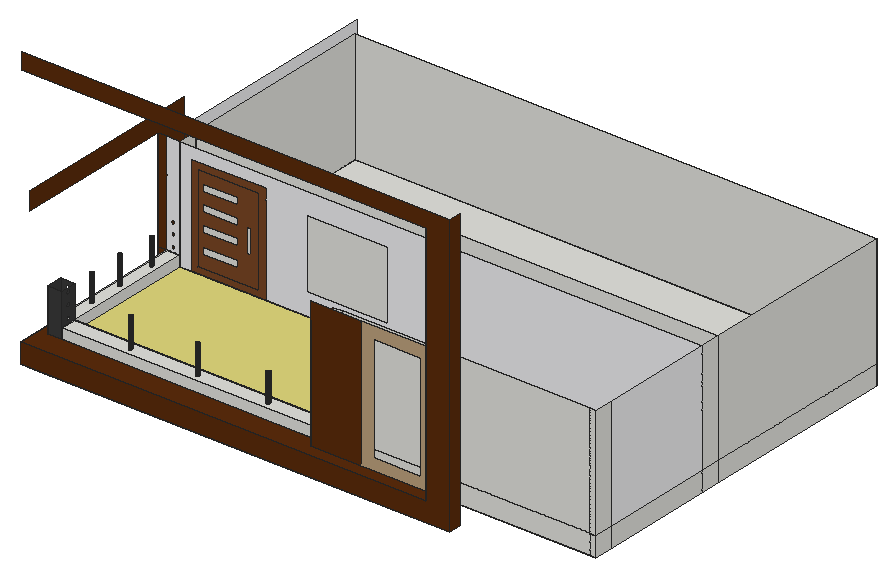
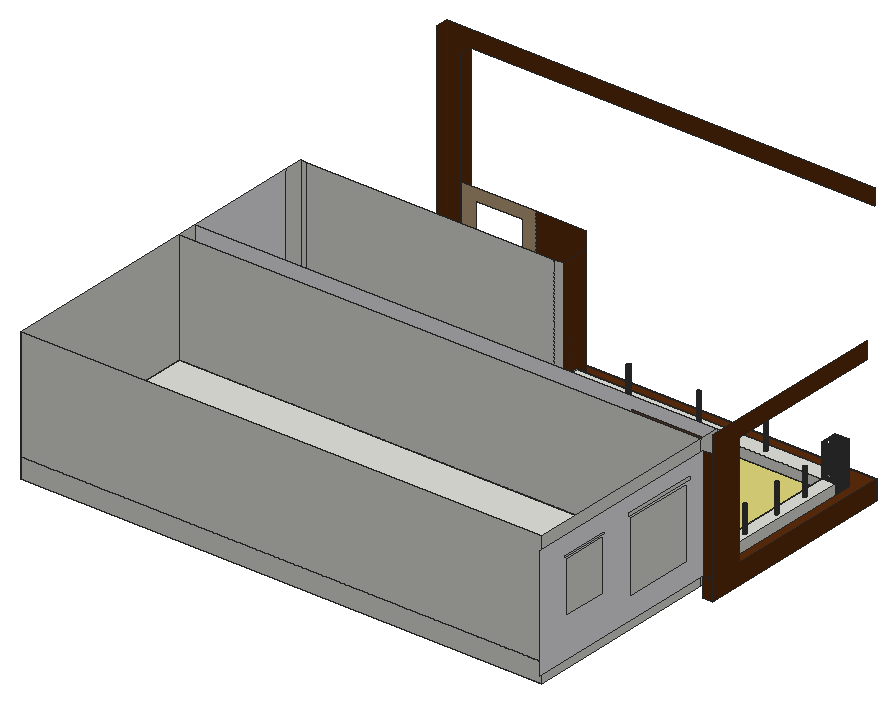
# SketchUp Ruby script. Lengths in inches.
U = 1.inch
M = Sketchup.active_model
def pt(a) = Geom::Point3d.new(a.map { |v| v * U })
def face(e, loops, mat)
  f = e.add_face(loops[0].map { |a| pt(a) })
  loops[1..].each { |l| e.add_face(l.map { |a| pt(a) }).erase! }
  f.material = f.back_material = mat if mat
  f
end
# faces: each face lists its corners as indices into pts; further lists are holes
def faces(e, pts, list, mat = nil) = list.each { |f| face(e, (f[0].is_a?(Array) ? f : [f]).map { |l| l.map { |i| pts[i] } }, mat) }
# xy, xz, yz: faces in a plane at the given z, y or x. An outline is a flat list of corners, or four numbers for a rectangle; further outlines are holes
def ring(l) = l.size == 4 ? [[l[0], l[1]], [l[2], l[1]], [l[2], l[3]], [l[0], l[3]]] : l.each_slice(2).to_a
def flat(e, list, mat, &to3) = list.each { |f| face(e, (f[0].is_a?(Array) ? f : [f]).map { |l| ring(l).map { |u, v| to3.(u, v) } }, mat) }
def xy(e, z, list, mat = nil) = flat(e, list, mat) { |x, y| [x, y, z] }
def xz(e, y, list, mat = nil) = flat(e, list, mat) { |x, z| [x, y, z] }
def yz(e, x, list, mat = nil) = flat(e, list, mat) { |y, z| [x, y, z] }
def lines(e, pts, list) = list.each { |a, b| e.add_line(pt(pts[a]), pt(pts[b])) }
# prism: a flat outline (further loops are holes) pulled along v
def prism(e, loops, v, mat = nil)
  f = face(e, loops, mat); d = Geom::Vector3d.new(v.map { |x| x * U })
  f.pushpull(f.normal.samedirection?(d) ? d.length : -d.length)
end
def box(e, o, s, mat = nil) = prism(e, [[o, [o[0] + s[0], o[1], o[2]], [o[0] + s[0], o[1] + s[1], o[2]], [o[0], o[1] + s[1], o[2]]]], [0, 0, s[2]], mat)
def at(x, y, z, deg = 0) = Geom::Transformation.translation(pt([x, y, z])) * Geom::Transformation.rotation(ORIGIN, Z_AXIS, deg.degrees)
def axes(o, x, y, z) = Geom::Transformation.new([*x, 0, *y, 0, *z, 0, *pt(o).to_a, 1])
def part(name) = M.definitions.add(name)
# library, detail: a bought-in or finely detailed component or shape, given as its bounding box
def library(name, o, s) = part(name).tap { |d| box(d.entities, o, s) }
def detail(e, o, s) = box(e.add_group.entities, o, s)
def put(e, d, t, mat = nil) = e.add_instance(d, t).tap { |i| i.material = mat if mat }
def group(e, t, mat = nil) = e.add_group.tap { |g| g.transformation = t; g.material = mat if mat }.entities
root = M.entities
M.materials.add("[0035_Tan]").color = [188, 161, 125]
M.materials.add("[0043_SaddleBrown]").color = [91, 44, 12]
M.materials.add("[Blinds Vertical Pattern]").color = [237, 237, 239]
M.materials.add("[Carpet Diamond Yellow]").color = [226, 217, 124]
M.materials.add("[Color M07]").color = [58, 58, 58]
M.materials.add("[Wood Veneer 01]").color = [120, 70, 37]
xy(root,621.625,[[85.98,538.2,560.26,556.28],[85.98,556.28,560.26,737.09]])
xy(root,621.625,[[65.42,382.09,73.92,393.34],[73.92,382.09,320.99,393.34],[320.99,382.09,456.39,393.34],[65.42,393.34,73.92,538.2],[65.42,538.2,73.92,568.32]],"[0043_SaddleBrown]")
xy(root,621.625,[[73.92,393.34,73.92,538.2,560.26,538.2,560.26,418.04,320.99,418.04,320.99,393.34]],"[Blinds Vertical Pattern]")
xy(root,639.5625,[[73.92,403.22,85.98,418.04],[85.98,403.22,320.99,418.04],[73.92,418.04,85.98,538.2],[85.98,538.2,560.26,556.28],[85.98,556.28,560.26,737.09]])
xy(root,639.5625,[[65.42,382.09,434.25,382.09,434.25,393.34,320.99,393.34,320.99,403.22,73.92,403.22,73.92,538.2,65.42,538.2]],"[0043_SaddleBrown]")
xy(root,639.5625,[[85.98,418.04,560.26,538.2]],"[Carpet Diamond Yellow]")
xy(root,648.75,[[[85.98,403.22,320.99,418.04],[142.95,408.99,142.55,409.04,142.17,409.2,141.85,409.45,141.6,409.77,141.44,410.15,141.39,410.55,141.44,410.96,141.6,411.34,141.85,411.66,142.17,411.91,142.55,412.0625,142.95,412.12,143.36,412.0625,143.73,411.91,144.06,411.66,144.3,411.34,144.46,410.96,144.51,410.55,144.46,410.15,144.3,409.77,144.06,409.45,143.73,409.2,143.36,409.04],[268.26,408.99,267.86,409.04,267.48,409.2,267.16,409.45,266.91,409.77,266.75,410.15,266.7,410.55,266.75,410.96,266.91,411.34,267.16,411.66,267.48,411.91,267.86,412.0625,268.26,412.12,268.67,412.0625,269.04,411.91,269.37,411.66,269.62,411.34,269.77,410.96,269.83,410.55,269.77,410.15,269.62,409.77,269.37,409.45,269.04,409.2,268.67,409.04],[204.26,408.99,203.86,409.04,203.48,409.2,203.16,409.45,202.91,409.77,202.75,410.15,202.7,410.55,202.75,410.96,202.91,411.34,203.16,411.66,203.48,411.91,203.86,412.0625,204.26,412.12,204.67,412.0625,205.04,411.91,205.37,411.66,205.62,411.34,205.77,410.96,205.83,410.55,205.77,410.15,205.62,409.77,205.37,409.45,205.04,409.2,204.67,409.04]],[142.95,408.99,142.55,409.04,142.17,409.2,141.85,409.45,141.6,409.77,141.44,410.15,141.39,410.55,141.44,410.96,141.6,411.34,141.85,411.66,142.17,411.91,142.55,412.0625,142.95,412.12,143.36,412.0625,143.73,411.91,144.06,411.66,144.3,411.34,144.46,410.96,144.51,410.55,144.46,410.15,144.3,409.77,144.06,409.45,143.73,409.2,143.36,409.04],[204.26,408.99,203.86,409.04,203.48,409.2,203.16,409.45,202.91,409.77,202.75,410.15,202.7,410.55,202.75,410.96,202.91,411.34,203.16,411.66,203.48,411.91,203.86,412.0625,204.26,412.12,204.67,412.0625,205.04,411.91,205.37,411.66,205.62,411.34,205.77,410.96,205.83,410.55,205.77,410.15,205.62,409.77,205.37,409.45,205.04,409.2,204.67,409.04],[268.26,408.99,267.86,409.04,267.48,409.2,267.16,409.45,266.91,409.77,266.75,410.15,266.7,410.55,266.75,410.96,266.91,411.34,267.16,411.66,267.48,411.91,267.86,412.0625,268.26,412.12,268.67,412.0625,269.04,411.91,269.37,411.66,269.62,411.34,269.77,410.96,269.83,410.55,269.77,410.15,269.62,409.77,269.37,409.45,269.04,409.2,268.67,409.04],[[73.92,418.04,85.98,538.2],[79.49,444.43,79.08,444.48,78.7,444.64,78.38,444.88,78.13,445.21,77.98,445.59,77.92,445.99,77.98,446.39,78.13,446.77,78.38,447.09,78.7,447.34,79.08,447.5,79.49,447.55,79.89,447.5,80.27,447.34,80.59,447.09,80.84,446.77,81,446.39,81.05,445.99,81,445.59,80.84,445.21,80.59,444.88,80.27,444.64,79.89,444.48],[79.49,512.61,79.08,512.67,78.7,512.82,78.38,513.07,78.13,513.4,77.98,513.77,77.92,514.18,77.98,514.58,78.13,514.96,78.38,515.28,78.7,515.53,79.08,515.6875,79.49,515.74,79.89,515.6875,80.27,515.53,80.59,515.28,80.84,514.96,81,514.58,81.05,514.18,81,513.77,80.84,513.4,80.59,513.07,80.27,512.82,79.89,512.67],[79.49,476.18,79.08,476.23,78.7,476.39,78.38,476.63,78.13,476.96,77.98,477.34,77.92,477.74,77.98,478.14,78.13,478.52,78.38,478.84,78.7,479.09,79.08,479.25,79.49,479.3,79.89,479.25,80.27,479.09,80.59,478.84,80.84,478.52,81,478.14,81.05,477.74,81,477.34,80.84,476.96,80.59,476.63,80.27,476.39,79.89,476.23]],
  [79.49,444.43,79.08,444.48,78.7,444.64,78.38,444.88,78.13,445.21,77.98,445.59,77.92,445.99,77.98,446.39,78.13,446.77,78.38,447.09,78.7,447.34,79.08,447.5,79.49,447.55,79.89,447.5,80.27,447.34,80.59,447.09,80.84,446.77,81,446.39,81.05,445.99,81,445.59,80.84,445.21,80.59,444.88,80.27,444.64,79.89,444.48],[79.49,476.18,79.08,476.23,78.7,476.39,78.38,476.63,78.13,476.96,77.98,477.34,77.92,477.74,77.98,478.14,78.13,478.52,78.38,478.84,78.7,479.09,79.08,479.25,79.49,479.3,79.89,479.25,80.27,479.09,80.59,478.84,80.84,478.52,81,478.14,81.05,477.74,81,477.34,80.84,476.96,80.59,476.63,80.27,476.39,79.89,476.23],[79.49,512.61,79.08,512.67,78.7,512.82,78.38,513.07,78.13,513.4,77.98,513.77,77.92,514.18,77.98,514.58,78.13,514.96,78.38,515.28,78.7,515.53,79.08,515.6875,79.49,515.74,79.89,515.6875,80.27,515.53,80.59,515.28,80.84,514.96,81,514.58,81.05,514.18,81,513.77,80.84,513.4,80.59,513.07,80.27,512.82,79.89,512.67]])
xz(root,382.09,[[65.42,621.625,456.39,621.625,456.39,876.375,66.61,876.375,66.61,861.625,434.25,861.625,434.25,639.5625,65.42,639.5625]],"[0043_SaddleBrown]")
xz(root,393.34,[[[366.56,639.5625,434.25,757.5],[378.18,649.8125,421.12,746.5625]]],"[0035_Tan]")
xz(root,393.34,[[320.99,639.5625,366.56,757.5]],"[0043_SaddleBrown]")
xz(root,403.22,[[85.98,639.5625,320.99,648.75]])
xz(root,403.22,[[73.92,639.5625,85.98,678.5625]],"[Color M07]")
xz(root,418.04,[[320.99,621.625,329.72,639.5625],[329.72,621.625,554.62,639.5625],[554.62,621.625,560.26,639.5625],[73.92,639.5625,85.98,648.75],[85.98,639.5625,320.99,648.75],
  [320.99,639.5625,329.72,741.625],[329.72,639.5625,554.62,741.625],[554.62,639.5625,560.26,741.625]])
xz(root,418.04,[[[73.92,648.75,85.98,678.5625],[79.68,671.45,80.15,671.51,80.58,671.6875,80.96,671.98,81.25,672.35,81.43,672.79,81.49,673.26,81.43,673.73,81.25,674.17,80.96,674.54,80.58,674.83,80.15,675.01,79.68,675.07,79.21,675.01,78.77,674.83,78.4,674.54,78.11,674.17,77.93,673.73,77.87,673.26,77.93,672.79,78.11,672.35,78.4,671.98,78.77,671.6875,79.21,671.51],[79.68,661.95,80.15,662.01,80.58,662.1875,80.96,662.48,81.25,662.85,81.43,663.29,81.49,663.76,81.43,664.23,81.25,664.67,80.96,665.04,80.58,665.33,80.15,665.51,79.68,665.57,79.21,665.51,78.77,665.33,78.4,665.04,78.11,664.67,77.93,664.23,77.87,663.76,77.93,663.29,78.11,662.85,78.4,662.48,78.77,662.1875,79.21,662.01],[79.68,651.2,80.15,651.26,80.58,651.4375,80.96,651.73,81.25,652.1,81.43,652.54,81.49,653.01,81.43,653.48,81.25,653.92,80.96,654.29,80.58,654.58,80.15,654.76,79.68,654.82,79.21,654.76,78.77,654.58,78.4,654.29,78.11,653.92,77.93,653.48,77.87,653.01,77.93,652.54,78.11,652.1,78.4,651.73,78.77,651.4375,79.21,651.26]]],"[Color M07]")
xz(root,538.2,[[85.98,621.625,560.26,639.5625],[73.92,639.5625,85.98,648.75]])
xz(root,538.2,[[65.42,639.5625,73.92,648.75],[65.42,648.75,73.92,741.625]],"[0043_SaddleBrown]")
xz(root,538.2,[[[85.98,639.5625,96.59,639.5625,96.59,730.6875,163.47,730.6875,163.47,639.5625,560.26,639.5625,560.26,741.625,85.98,741.625],[201.38,659.52,275.19,722.4]],[[73.92,648.75,85.98,741.625],[79.68,651.2,79.21,651.26,78.77,651.4375,78.4,651.73,78.11,652.1,77.93,652.54,77.87,653.01,77.93,653.48,78.11,653.92,78.4,654.29,78.77,654.58,79.21,654.76,79.68,654.82,80.15,654.76,80.58,654.58,80.96,654.29,81.25,653.92,81.43,653.48,81.49,653.01,81.43,652.54,81.25,652.1,80.96,651.73,80.58,651.4375,80.15,651.26],[79.68,661.95,79.21,662.01,78.77,662.1875,78.4,662.48,78.11,662.85,77.93,663.29,77.87,663.76,77.93,664.23,78.11,664.67,78.4,665.04,78.77,665.33,79.21,665.51,79.68,665.57,80.15,665.51,80.58,665.33,80.96,665.04,81.25,664.67,81.43,664.23,81.49,663.76,81.43,663.29,81.25,662.85,80.96,662.48,80.58,662.1875,80.15,662.01],[79.68,671.45,79.21,671.51,78.77,671.6875,78.4,671.98,78.11,672.35,77.93,672.79,77.87,673.26,77.93,673.73,78.11,674.17,78.4,674.54,78.77,674.83,79.21,675.01,79.68,675.07,80.15,675.01,80.58,674.83,80.96,674.54,81.25,674.17,81.43,673.73,81.49,673.26,81.43,672.79,81.25,672.35,80.96,671.98,80.58,671.6875,80.15,671.51]]],"[Blinds Vertical Pattern]")
xz(root,538.2,[[[96.59,639.5625,163.47,730.6875],[102.17,645.14,157.89,725.11]],[[102.17,645.14,157.89,725.11],[106.93,707.84,137.99,714.4],[106.93,656.78,137.99,663.34],[106.93,691.28,137.99,697.84],[106.93,674.53,137.99,681.09],[146.5,671.28,150.06,692.91]]],"[Wood Veneer 01]")
xz(root,556.28,[[85.98,621.625,560.26,639.5625],[85.98,639.5625,560.26,741.625]])
xz(root,568.32,[[65.42,621.625,73.92,639.5625],[65.42,639.5625,73.92,741.625]],"[0043_SaddleBrown]")
xz(root,737.09,[[85.98,621.625,560.26,639.5625],[85.98,639.5625,560.26,741.625]])
yz(root,65.42,[[382.09,621.625,382.09,639.5625,538.2,639.5625,538.2,741.625,393.34,741.625,393.34,757.5,568.32,757.5,568.32,621.625]],"[0043_SaddleBrown]")
yz(root,73.92,[[418.04,639.5625,538.2,648.75]])
yz(root,73.92,[[[568.32,639.5625,753.91,741.625],[587.21,659.05,651.27,723.11],[682.92,675.28,724.55,722.34],[582.96,724.34,654.15,728.22],[680.2,723.29,726.88,725.66]]],"[Blinds Vertical Pattern]")
yz(root,73.92,[[403.22,639.5625,418.04,678.5625]],"[Color M07]")
yz(root,85.98,[[538.2,621.625,556.28,639.5625],[556.28,621.625,737.09,639.5625],[403.22,639.5625,418.04,648.75],[418.04,639.5625,538.2,648.75],[538.2,639.5625,556.28,741.625],
  [556.28,639.5625,737.09,741.625]])
yz(root,85.98,[[[403.22,648.75,418.04,678.5625],[410.75,651.38,410.22,651.45,409.72,651.66,409.29,651.99,408.97,652.41,408.76,652.91,408.6875,653.44,408.76,653.98,408.97,654.48,409.29,654.9,409.72,655.23,410.22,655.4375,410.75,655.51,411.29,655.4375,411.78,655.23,412.21,654.9,412.54,654.48,412.74,653.98,412.8125,653.44,412.74,652.91,412.54,652.41,412.21,651.99,411.78,651.66,411.29,651.45],[410.75,662.32,410.22,662.39,409.72,662.6,409.29,662.92,408.97,663.35,408.76,663.85,408.6875,664.38,408.76,664.92,408.97,665.41,409.29,665.84,409.72,666.17,410.22,666.375,410.75,666.44,411.29,666.375,411.78,666.17,412.21,665.84,412.54,665.41,412.74,664.92,412.8125,664.38,412.74,663.85,412.54,663.35,412.21,662.92,411.78,662.6,411.29,662.39],[410.75,672.82,410.22,672.89,409.72,673.1,409.29,673.42,408.97,673.85,408.76,674.35,408.6875,674.88,408.76,675.42,408.97,675.91,409.29,676.34,409.72,676.67,410.22,676.875,410.75,676.94,411.29,676.875,411.78,676.67,412.21,676.34,412.54,675.91,412.74,675.42,412.8125,674.88,412.74,674.35,412.54,673.85,412.21,673.42,411.78,673.1,411.29,672.89]]],"[Color M07]")
yz(root,320.99,[[403.22,639.5625,418.04,648.75]])
yz(root,320.99,[[[393.34,639.5625,393.34,741.625,418.04,741.625,418.04,648.75,403.22,648.75,403.22,639.5625],[410.75,662.32,411.29,662.39,411.78,662.6,412.21,662.92,412.54,663.35,412.74,663.85,412.8125,664.38,412.74,664.92,412.54,665.41,412.21,665.84,411.78,666.17,411.29,666.375,410.75,666.44,410.22,666.375,409.72,666.17,409.29,665.84,408.97,665.41,408.76,664.92,408.6875,664.38,408.76,663.85,408.97,663.35,409.29,662.92,409.72,662.6,410.22,662.39],[410.75,651.38,411.29,651.45,411.78,651.66,412.21,651.99,412.54,652.41,412.74,652.91,412.8125,653.44,412.74,653.98,412.54,654.48,412.21,654.9,411.78,655.23,411.29,655.4375,410.75,655.51,410.22,655.4375,409.72,655.23,409.29,654.9,408.97,654.48,408.76,653.98,408.6875,653.44,408.76,652.91,408.97,652.41,409.29,651.99,409.72,651.66,410.22,651.45],[410.75,672.82,411.29,672.89,411.78,673.1,412.21,673.42,412.54,673.85,412.74,674.35,412.8125,674.88,412.74,675.42,412.54,675.91,412.21,676.34,411.78,676.67,411.29,676.875,410.75,676.94,410.22,676.875,409.72,676.67,409.29,676.34,408.97,675.91,408.76,675.42,408.6875,674.88,408.76,674.35,408.97,673.85,409.29,673.42,409.72,673.1,410.22,672.89]]],"[0043_SaddleBrown]")
yz(root,434.25,[[382.09,639.5625,393.34,861.625]],"[0043_SaddleBrown]")
yz(root,456.39,[[382.09,621.625,393.34,876.375]],"[0043_SaddleBrown]")
yz(root,560.26,[[418.04,621.625,434.85,639.5625],[434.85,621.625,538.2,639.5625],[538.2,621.625,556.28,639.5625],[556.28,621.625,737.09,639.5625],[418.04,639.5625,434.85,741.625],
  [538.2,639.5625,556.28,741.625],[556.28,639.5625,737.09,741.625]])
yz(root,560.26,[[434.85,639.5625,538.2,741.625]],"[Blinds Vertical Pattern]")
p = [[142.17,409.2,648.75],[142.55,409.04,648.75],[142.55,409.04,675.42],[142.17,409.2,675.42],[142.95,408.99,648.75],[142.95,408.99,675.42],
  [143.36,409.04,648.75],[143.36,409.04,675.42],[143.73,409.2,648.75],[143.73,409.2,675.42],[203.48,409.2,648.75],[203.86,409.04,648.75],
  [203.86,409.04,674.88],[203.48,409.2,674.88],[204.26,408.99,648.75],[204.26,408.99,674.88],[204.67,409.04,648.75],[204.67,409.04,674.88],
  [205.04,409.2,648.75],[205.04,409.2,674.88],[267.48,409.2,648.75],[267.86,409.04,648.75],[267.86,409.04,674.1875],[267.48,409.2,674.1875],
  [268.26,408.99,648.75],[268.26,408.99,674.1875],[268.67,409.04,648.75],[268.67,409.04,674.1875],[269.04,409.2,648.75],[269.04,409.2,674.1875],
  [141.85,409.45,648.75],[141.85,409.45,675.42],[144.06,409.45,648.75],[144.06,409.45,675.42],[203.16,409.45,648.75],[203.16,409.45,674.88],
  [205.37,409.45,648.75],[205.37,409.45,674.88],[267.16,409.45,648.75],[267.16,409.45,674.1875],[269.37,409.45,648.75],[269.37,409.45,674.1875],
  [141.6,409.77,648.75],[141.6,409.77,675.42],[144.3,409.77,648.75],[144.3,409.77,675.42],[202.91,409.77,648.75],[202.91,409.77,674.88],
  [205.62,409.77,648.75],[205.62,409.77,674.88],[266.91,409.77,648.75],[266.91,409.77,674.1875],[269.62,409.77,648.75],[269.62,409.77,674.1875],
  [141.44,410.15,648.75],[141.44,410.15,675.42],[144.46,410.15,648.75],[144.46,410.15,675.42],[202.75,410.15,648.75],[202.75,410.15,674.88],
  [205.77,410.15,648.75],[205.77,410.15,674.88],[266.75,410.15,648.75],[266.75,410.15,674.1875],[269.77,410.15,648.75],[269.77,410.15,674.1875],
  [141.39,410.55,648.75],[141.39,410.55,675.42],[144.51,410.55,648.75],[144.51,410.55,675.42],[202.7,410.55,648.75],[202.7,410.55,674.88],
  [205.83,410.55,648.75],[205.83,410.55,674.88],[266.7,410.55,648.75],[266.7,410.55,674.1875],[269.83,410.55,648.75],[269.83,410.55,674.1875],
  [141.44,410.96,648.75],[141.44,410.96,675.42],[144.46,410.96,648.75],[144.46,410.96,675.42],[202.75,410.96,648.75],[202.75,410.96,674.88],
  [205.77,410.96,648.75],[205.77,410.96,674.88],[266.75,410.96,648.75],[266.75,410.96,674.1875],[269.77,410.96,648.75],[269.77,410.96,674.1875],
  [141.6,411.34,648.75],[141.6,411.34,675.42],[144.3,411.34,648.75],[144.3,411.34,675.42],[202.91,411.34,648.75],[202.91,411.34,674.88],
  [205.62,411.34,648.75],[205.62,411.34,674.88],[266.91,411.34,648.75],[266.91,411.34,674.1875],[269.62,411.34,648.75],[269.62,411.34,674.1875],
  [141.85,411.66,648.75],[141.85,411.66,675.42],[144.06,411.66,648.75],[144.06,411.66,675.42],[203.16,411.66,648.75],[203.16,411.66,674.88],
  [205.37,411.66,648.75],[205.37,411.66,674.88],[267.16,411.66,648.75],[267.16,411.66,674.1875],[269.37,411.66,648.75],[269.37,411.66,674.1875],
  [142.17,411.91,648.75],[142.17,411.91,675.42],[143.73,411.91,648.75],[143.73,411.91,675.42],[203.48,411.91,648.75],[203.48,411.91,674.88],
  [205.04,411.91,648.75],[205.04,411.91,674.88],[267.48,411.91,648.75],[267.48,411.91,674.1875],[269.04,411.91,648.75],[269.04,411.91,674.1875],
  [142.55,412.0625,648.75],[142.55,412.0625,675.42],[143.36,412.0625,648.75],[143.36,412.0625,675.42],[203.86,412.0625,648.75],[203.86,412.0625,674.88],
  [204.67,412.0625,648.75],[204.67,412.0625,674.88],[267.86,412.0625,648.75],[267.86,412.0625,674.1875],[268.67,412.0625,648.75],[268.67,412.0625,674.1875],
  [142.95,412.12,648.75],[142.95,412.12,675.42],[204.26,412.12,648.75],[204.26,412.12,674.88],[268.26,412.12,648.75],[268.26,412.12,674.1875],
  [79.08,444.48,648.75],[79.49,444.43,648.75],[79.49,444.43,672.79],[79.08,444.48,672.79],[79.89,444.48,648.75],[79.89,444.48,672.79],
  [78.7,444.64,648.75],[78.7,444.64,672.79],[80.27,444.64,648.75],[80.27,444.64,672.79],[78.38,444.88,648.75],[78.38,444.88,672.79],
  [80.59,444.88,648.75],[80.59,444.88,672.79],[78.13,445.21,648.75],[78.13,445.21,672.79],[80.84,445.21,648.75],[80.84,445.21,672.79],
  [77.98,445.59,648.75],[77.98,445.59,672.79],[81,445.59,648.75],[81,445.59,672.79],[77.92,445.99,648.75],[77.93,445.96,672.79],
  [77.92,445.99,672.79],[81.05,445.99,648.75],[81.05,445.99,672.79],[77.98,446.39,648.75],[77.93,446.02,672.79],[77.98,446.39,672.79],
  [81,446.39,648.75],[81,446.39,672.79],[78.13,446.77,648.75],[78.13,446.77,672.79],[80.84,446.77,648.75],[80.84,446.77,672.79],
  [78.38,447.09,648.75],[78.38,447.09,672.79],[80.59,447.09,648.75],[80.59,447.09,672.79],[78.7,447.34,648.75],[78.7,447.34,672.79],
  [80.27,447.34,648.75],[80.27,447.34,672.79],[79.08,447.5,648.75],[79.08,447.5,672.79],[79.89,447.5,648.75],[79.89,447.5,672.79],
  [79.49,447.55,648.75],[79.49,447.55,672.79],[78.7,476.39,648.75],[79.08,476.23,648.75],[79.08,476.23,674.0625],[78.7,476.39,674.0625],
  [79.49,476.18,648.75],[79.49,476.18,674.0625],[79.89,476.23,648.75],[79.89,476.23,674.0625],[80.27,476.39,648.75],[80.27,476.39,674.0625],
  [78.38,476.63,648.75],[78.38,476.63,674.0625],[80.59,476.63,648.75],[80.59,476.63,674.0625],[78.13,476.96,648.75],[78.13,476.96,674.0625],
  [80.84,476.96,648.75],[80.84,476.96,674.0625],[77.98,477.34,648.75],[77.98,477.34,674.0625],[81,477.34,648.75],[81,477.34,674.0625],
  [77.92,477.74,648.75],[77.92,477.74,674.0625],[81.05,477.74,648.75],[81.05,477.74,674.0625],[77.98,478.14,648.75],[77.98,478.14,674.0625],
  [81,478.14,648.75],[81,478.14,674.0625],[78.13,478.52,648.75],[78.13,478.52,674.0625],[80.84,478.52,648.75],[80.84,478.52,674.0625],
  [78.38,478.84,648.75],[78.38,478.84,674.0625],[80.59,478.84,648.75],[80.59,478.84,674.0625],[78.7,479.09,648.75],[78.7,479.09,674.0625],
  [80.27,479.09,648.75],[80.27,479.09,674.0625],[79.08,479.25,648.75],[79.08,479.25,674.0625],[79.89,479.25,648.75],[79.89,479.25,674.0625],
  [79.49,479.3,648.75],[79.49,479.3,674.0625],[79.08,512.67,648.75],[79.49,512.61,648.75],[79.49,512.61,672.3125],[79.08,512.67,672.3125],
  [79.89,512.67,648.75],[79.89,512.67,672.3125],[78.7,512.82,648.75],[78.7,512.82,672.3125],[80.27,512.82,648.75],[80.27,512.82,672.3125],
  [78.38,513.07,648.75],[78.38,513.07,672.3125],[80.59,513.07,648.75],[80.59,513.07,672.3125],[78.13,513.4,648.75],[78.13,513.4,672.3125],
  [80.84,513.4,648.75],[80.84,513.4,672.3125],[77.98,513.77,648.75],[77.98,513.77,672.3125],[81,513.77,648.75],[81,513.77,672.3125],
  [77.92,514.18,648.75],[77.92,514.18,672.3125],[81.05,514.18,648.75],[81.05,514.18,672.3125],[77.98,514.58,648.75],[77.98,514.58,672.3125],
  [81,514.58,648.75],[81,514.58,672.3125],[78.13,514.96,648.75],[78.13,514.96,672.3125],[80.84,514.96,648.75],[80.84,514.96,672.3125],
  [78.38,515.28,648.75],[78.38,515.28,672.3125],[80.59,515.28,648.75],[80.59,515.28,672.3125],[78.7,515.53,648.75],[78.7,515.53,672.3125],
  [80.27,515.53,648.75],[80.27,515.53,672.3125],[79.08,515.6875,648.75],[79.08,515.6875,672.3125],[79.89,515.6875,648.75],[79.89,515.6875,672.3125],
  [79.49,515.74,648.75],[79.49,515.74,672.3125]]
faces(root,p,[[0,1,2,3],[1,4,5,2],[4,6,7,5],[6,8,9,7],[10,11,12,13],[11,14,15,12],[14,16,17,15],[16,18,19,17],
  [20,21,22,23],[21,24,25,22],[24,26,27,25],[26,28,29,27],[30,0,3,31],[8,32,33,9],[34,10,13,35],[18,36,37,19],
  [38,20,23,39],[28,40,41,29],[42,30,31,43],[32,44,45,33],[46,34,35,47],[36,48,49,37],[50,38,39,51],[40,52,53,41],
  [54,42,43,55],[44,56,57,45],[58,46,47,59],[48,60,61,49],[62,50,51,63],[52,64,65,53],[66,54,55,67],[56,68,69,57],
  [70,58,59,71],[60,72,73,61],[74,62,63,75],[64,76,77,65],[78,66,67,79],[68,80,81,69],[82,70,71,83],[72,84,85,73],
  [86,74,75,87],[76,88,89,77],[90,78,79,91],[80,92,93,81],[94,82,83,95],[84,96,97,85],[98,86,87,99],[88,100,101,89],
  [102,90,91,103],[92,104,105,93],[106,94,95,107],[96,108,109,97],[110,98,99,111],[100,112,113,101],[114,102,103,115],[104,116,117,105],
  [118,106,107,119],[108,120,121,109],[122,110,111,123],[112,124,125,113],[126,114,115,127],[116,128,129,117],[130,118,119,131],[120,132,133,121],
  [134,122,123,135],[124,136,137,125],[138,126,127,139],[128,138,139,129],[140,130,131,141],[132,140,141,133],[142,134,135,143],[136,142,143,137],
  [144,145,146,147],[145,148,149,146],[150,144,147,151],[148,152,153,149],[154,150,151,155],[152,156,157,153],[158,154,155,159],[156,160,161,157],
  [162,158,159,163],[160,164,165,161],[166,162,163,167,168],[164,169,170,165],[171,166,168,172,173],[169,174,175,170],[176,171,173,177],[174,178,179,175],
  [180,176,177,181],[178,182,183,179],[184,180,181,185],[182,186,187,183],[188,184,185,189],[186,190,191,187],[192,188,189,193],[190,192,193,191],
  [194,195,196,197],[195,198,199,196],[198,200,201,199],[200,202,203,201],[204,194,197,205],[202,206,207,203],[208,204,205,209],[206,210,211,207],
  [212,208,209,213],[210,214,215,211],[216,212,213,217],[214,218,219,215],[220,216,217,221],[218,222,223,219],[224,220,221,225],[222,226,227,223],
  [228,224,225,229],[226,230,231,227],[232,228,229,233],[230,234,235,231],[236,232,233,237],[234,238,239,235],[240,236,237,241],[238,240,241,239],
  [242,243,244,245],[243,246,247,244],[248,242,245,249],[246,250,251,247],[252,248,249,253],[250,254,255,251],[256,252,253,257],[254,258,259,255],
  [260,256,257,261],[258,262,263,259],[264,260,261,265],[262,266,267,263],[268,264,265,269],[266,270,271,267],[272,268,269,273],[270,274,275,271],
  [276,272,273,277],[274,278,279,275],[280,276,277,281],[278,282,283,279],[284,280,281,285],[282,286,287,283],[288,284,285,289],[286,288,289,287]],"[Color M07]")
